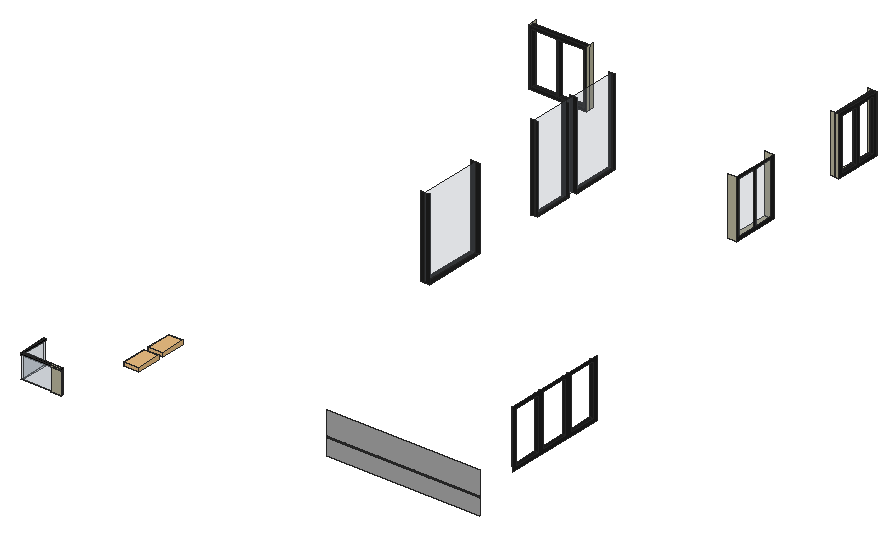
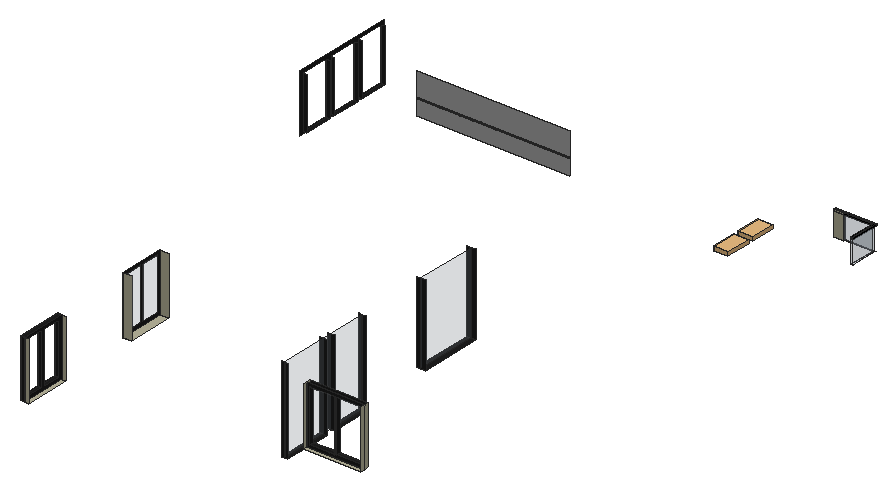
# SketchUp Ruby script. Lengths in inches.
U = 1.inch
M = Sketchup.active_model
def pt(a) = Geom::Point3d.new(a.map { |v| v * U })
def face(e, loops, mat)
  f = e.add_face(loops[0].map { |a| pt(a) })
  loops[1..].each { |l| e.add_face(l.map { |a| pt(a) }).erase! }
  f.material = f.back_material = mat if mat
  f
end
# faces: each face lists its corners as indices into pts; further lists are holes
def faces(e, pts, list, mat = nil) = list.each { |f| face(e, (f[0].is_a?(Array) ? f : [f]).map { |l| l.map { |i| pts[i] } }, mat) }
# xy, xz, yz: faces in a plane at the given z, y or x. An outline is a flat list of corners, or four numbers for a rectangle; further outlines are holes
def ring(l) = l.size == 4 ? [[l[0], l[1]], [l[2], l[1]], [l[2], l[3]], [l[0], l[3]]] : l.each_slice(2).to_a
def flat(e, list, mat, &to3) = list.each { |f| face(e, (f[0].is_a?(Array) ? f : [f]).map { |l| ring(l).map { |u, v| to3.(u, v) } }, mat) }
def xy(e, z, list, mat = nil) = flat(e, list, mat) { |x, y| [x, y, z] }
def xz(e, y, list, mat = nil) = flat(e, list, mat) { |x, z| [x, y, z] }
def yz(e, x, list, mat = nil) = flat(e, list, mat) { |y, z| [x, y, z] }
def lines(e, pts, list) = list.each { |a, b| e.add_line(pt(pts[a]), pt(pts[b])) }
# prism: a flat outline (further loops are holes) pulled along v
def prism(e, loops, v, mat = nil)
  f = face(e, loops, mat); d = Geom::Vector3d.new(v.map { |x| x * U })
  f.pushpull(f.normal.samedirection?(d) ? d.length : -d.length)
end
def box(e, o, s, mat = nil) = prism(e, [[o, [o[0] + s[0], o[1], o[2]], [o[0] + s[0], o[1] + s[1], o[2]], [o[0], o[1] + s[1], o[2]]]], [0, 0, s[2]], mat)
def at(x, y, z, deg = 0) = Geom::Transformation.translation(pt([x, y, z])) * Geom::Transformation.rotation(ORIGIN, Z_AXIS, deg.degrees)
def axes(o, x, y, z) = Geom::Transformation.new([*x, 0, *y, 0, *z, 0, *pt(o).to_a, 1])
def part(name) = M.definitions.add(name)
# library, detail: a bought-in or finely detailed component or shape, given as its bounding box
def library(name, o, s) = part(name).tap { |d| box(d.entities, o, s) }
def detail(e, o, s) = box(e.add_group.entities, o, s)
def put(e, d, t, mat = nil) = e.add_instance(d, t).tap { |i| i.material = mat if mat }
def group(e, t, mat = nil) = e.add_group.tap { |g| g.transformation = t; g.material = mat if mat }.entities
root = M.entities
M.materials.add("Concrete_04_1K").color = [184, 181, 156]
M.materials.add("D02_Buttercup_Glow").color = [255, 229, 155]
M.materials.add("Glass_Basic_01").color = [161, 173, 186]
M.materials["Glass_Basic_01"].alpha = 0.25
M.materials.add("M03_Pewter_Shine").color = [168, 168, 168]
M.materials.add("M07_Charcoal_Gleam").color = [58, 58, 58]
M.materials.add("M08_Obsidian_Black").color = [30, 30, 30]
M.materials.add("M09_Shadow_Night").color = [0, 0, 0]
c1 = part("Group\#59")
detail(c1.entities,[0,0,0],[15.125,26.3125,4])
xy(root,16,[[4462.07,3609.04,4472.4375,3609.73]],"Concrete_04_1K")
xy(root,16,[[4430.07,3609.04,4462.07,3609.73],[4430.07,3609.73,4430.76,3639.11],[4430.76,3609.73,4430.76,3639.11,4432.07,3639.11,4432.07,3611.04,4472.4375,3611.04,4472.4375,3609.73]],"Glass_Basic_01")
xy(root,18.55,[[4584.8125,4077.51,4588.3125,4117.75],[4588.3125,4077.51,4591.8125,4117.75],[4584.8125,4127.84,4588.3125,4177.75],[4588.3125,4127.84,4591.8125,4177.75]],"M08_Obsidian_Black")
xy(root,20.93,[[4586.8125,3932.41,4591.3125,3997.24],[4591.3125,3932.41,4595.8125,3997.24]],"M08_Obsidian_Black")
xy(root,40,[[4462.07,3609.04,4472.4375,3609.73]],"Concrete_04_1K")
xy(root,40,[[4430.07,3609.04,4462.07,3609.73],[4430.07,3609.73,4430.76,3639.11]],"Glass_Basic_01")
xy(root,40,[[4430.76,3609.73,4430.76,3639.11,4432.07,3639.11,4432.07,3611.04,4472.4375,3611.04,4472.4375,3609.73]],"M09_Shadow_Night")
xy(root,41.8125,[[4462.07,3609.04,4472.4375,3611.04]],"Concrete_04_1K")
xy(root,41.8125,[[4430.07,3609.04,4462.07,3609.04,4462.07,3611.04,4432.07,3611.04,4432.07,3639.11,4430.07,3639.11]],"M09_Shadow_Night")
xy(root,51,[[4769.8125,4101.42,4778.8125,4149.42],[4489.8125,4193.04,4549.8125,4197.54],[4489.8125,4197.54,4549.8125,4202.04],[4769.8125,4234.61,4778.8125,4282.61]],"Concrete_04_1K")
xy(root,54,[[4870.8125,3694.73,4874.8125,3724.73],[4870.8125,3730.73,4874.8125,3760.73],[4870.8125,3766.73,4874.8125,3796.73],[4492.8125,4193.04,4518.8125,4197.54],[4520.8125,4193.04,4546.8125,4197.54]],"M08_Obsidian_Black")
xz(root,3609.04,[[4462.07,40,4472.4375,41.8125]],"Concrete_04_1K")
xz(root,3609.04,[[4430.07,40,4462.07,41.8125]],"M09_Shadow_Night")
xz(root,3609.73,[[4462.07,16,4472.4375,40]],"Concrete_04_1K")
xz(root,3609.73,[[4430.76,16,4462.07,40]],"Glass_Basic_01")
xz(root,3611.04,[[4462.07,16,4472.4375,40],[4462.07,40,4472.4375,41.8125]],"Concrete_04_1K")
xz(root,3611.04,[[4432.07,16,4462.07,40]],"Glass_Basic_01")
xz(root,3611.04,[[4432.07,40,4462.07,41.8125]],"M09_Shadow_Night")
xz(root,3639.11,[[4430.76,16,4432.07,40]],"Glass_Basic_01")
xz(root,3639.11,[[4430.07,40,4432.07,41.8125]],"M09_Shadow_Night")
xz(root,3666.98,[[4701.3125,16,4860.07,32],[4701.3125,34,4860.07,58]],"M03_Pewter_Shine")
xz(root,3666.98,[[4701.3125,32,4860.07,34]],"M07_Charcoal_Gleam")
xz(root,3694.73,[[4870.8125,54,4874.8125,108]],"M08_Obsidian_Black")
xz(root,3724.73,[[4870.8125,54,4874.8125,108]],"M08_Obsidian_Black")
xz(root,3730.73,[[4870.8125,54,4874.8125,108]],"M08_Obsidian_Black")
xz(root,3760.73,[[4870.8125,54,4874.8125,108]],"M08_Obsidian_Black")
xz(root,3766.73,[[4870.8125,54,4874.8125,108]],"M08_Obsidian_Black")
xz(root,3796.73,[[4870.8125,54,4874.8125,108]],"M08_Obsidian_Black")
xz(root,3932.41,[[4586.8125,20.93,4591.3125,105.07],[4591.3125,20.93,4595.8125,105.07]],"M08_Obsidian_Black")
xz(root,3997.24,[[4586.8125,20.93,4591.3125,105.07],[4591.3125,20.93,4595.8125,105.07]],"M08_Obsidian_Black")
xz(root,4077.51,[[4584.8125,18.55,4588.3125,107.45],[4588.3125,18.55,4591.8125,107.45]],"M08_Obsidian_Black")
xz(root,4101.42,[[4769.8125,51,4778.8125,111]],"Concrete_04_1K")
xz(root,4117.75,[[4584.8125,18.55,4591.8125,107.45]],"M08_Obsidian_Black")
xz(root,4127.84,[[4584.8125,18.55,4591.8125,107.45]],"M08_Obsidian_Black")
xz(root,4149.42,[[4769.8125,51,4778.8125,111]],"Concrete_04_1K")
xz(root,4177.75,[[4584.8125,18.55,4588.3125,107.45],[4588.3125,18.55,4591.8125,107.45]],"M08_Obsidian_Black")
xz(root,4193.04,[[[4489.8125,51,4549.8125,111],[4492.8125,54,4518.8125,108],[4520.8125,54,4546.8125,108]]],"M08_Obsidian_Black")
xz(root,4197.54,[[[4489.8125,51,4549.8125,111],[4492.8125,54,4518.8125,108],[4520.8125,54,4546.8125,108]]],"M08_Obsidian_Black")
xz(root,4234.61,[[4769.8125,51,4778.8125,111]],"Concrete_04_1K")
xz(root,4282.61,[[4769.8125,51,4778.8125,111]],"Concrete_04_1K")
yz(root,4430.07,[[3609.04,40,3639.11,41.8125]],"M09_Shadow_Night")
yz(root,4430.76,[[3609.73,16,3639.11,40]],"Glass_Basic_01")
yz(root,4432.07,[[3611.04,16,3639.11,40]],"Glass_Basic_01")
yz(root,4432.07,[[3611.04,40,3639.11,41.8125]],"M09_Shadow_Night")
yz(root,4472.4375,[[3609.73,16,3611.04,40]],"Glass_Basic_01")
yz(root,4472.4375,[[3609.04,40,3611.04,41.8125]],"M09_Shadow_Night")
yz(root,4489.8125,[[4193.04,51,4197.54,111],[4197.54,51,4202.04,111]],"Concrete_04_1K")
yz(root,4492.8125,[[4193.04,54,4197.54,108]],"M08_Obsidian_Black")
yz(root,4518.8125,[[4193.04,54,4197.54,108]],"M08_Obsidian_Black")
yz(root,4520.8125,[[4193.04,54,4197.54,108]],"M08_Obsidian_Black")
yz(root,4546.8125,[[4193.04,54,4197.54,108]],"M08_Obsidian_Black")
yz(root,4549.8125,[[4193.04,51,4197.54,111],[4197.54,51,4202.04,111]],"Concrete_04_1K")
yz(root,4591.3125,[[3932.41,20.93,3997.24,105.07]],"Glass_Basic_01")
yz(root,4874.8125,[[[3691.73,51,3799.73,111],[3766.73,54,3796.73,108],[3730.73,54,3760.73,108],[3694.73,54,3724.73,108]]],"M08_Obsidian_Black")
g1 = group(root,at(4588.3125,4077.51,18.55),"Glass_Basic_01")
yz(g1,0,[[0,0,100.23,88.9]])
put(root,c1,at(4499.92,3655.87,33.0625),"D02_Buttercup_Glow")
put(root,c1,at(4499.92,3687.43,33.0625),"D02_Buttercup_Glow")
g2 = group(root,at(4778.8125,4234.61,51))
prism(g2,[[[0,0,0],[0,48,0],[0,48,60],[0,0,60]],[[0,25,3],[0,25,57],[0,45,57],[0,45,3]],[[0,3,57],[0,23,57],[0,23,3],[0,3,3]]],[-4.375,0,0],"M08_Obsidian_Black")
g3 = group(root,at(4778.8125,4101.42,51))
yz(g3,0,[[3,3,23,57],[25,3,45,57]],"Glass_Basic_01")
yz(g3,0,[[[0,0,48,60],[3,3,23,57],[25,3,45,57]]],"M08_Obsidian_Black")
